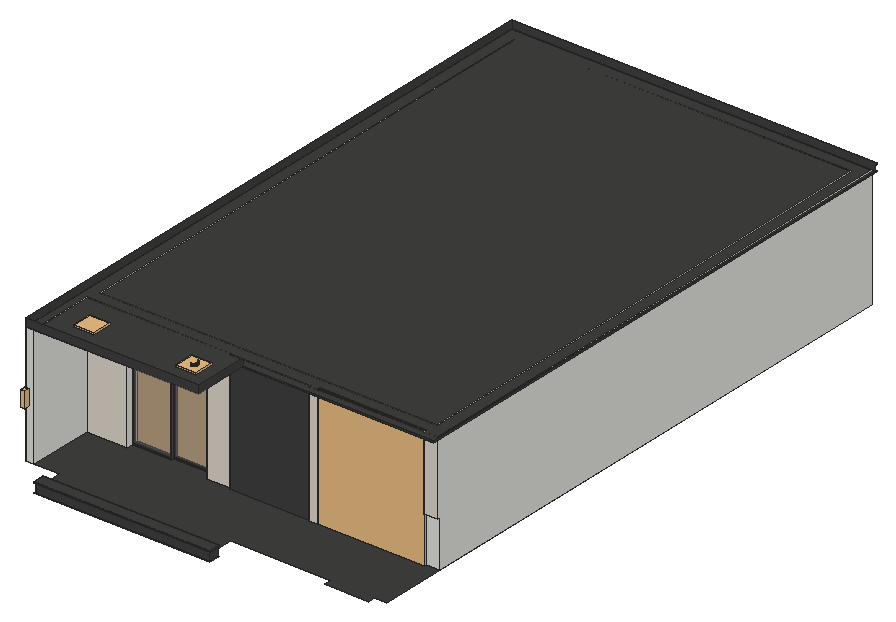
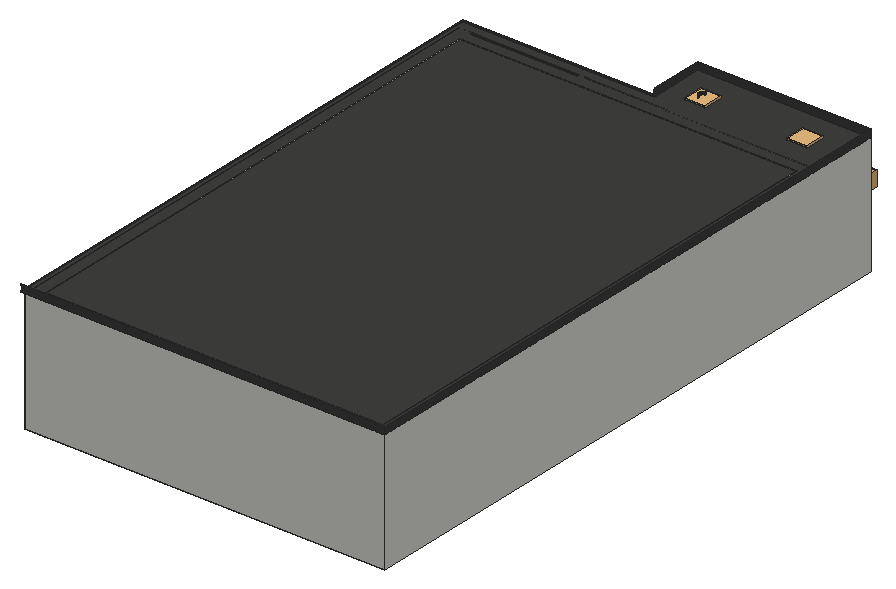
# SketchUp Ruby script. Lengths in inches.
U = 1.inch
M = Sketchup.active_model
def pt(a) = Geom::Point3d.new(a.map { |v| v * U })
def face(e, loops, mat)
  f = e.add_face(loops[0].map { |a| pt(a) })
  loops[1..].each { |l| e.add_face(l.map { |a| pt(a) }).erase! }
  f.material = f.back_material = mat if mat
  f
end
# faces: each face lists its corners as indices into pts; further lists are holes
def faces(e, pts, list, mat = nil) = list.each { |f| face(e, (f[0].is_a?(Array) ? f : [f]).map { |l| l.map { |i| pts[i] } }, mat) }
# xy, xz, yz: faces in a plane at the given z, y or x. An outline is a flat list of corners, or four numbers for a rectangle; further outlines are holes
def ring(l) = l.size == 4 ? [[l[0], l[1]], [l[2], l[1]], [l[2], l[3]], [l[0], l[3]]] : l.each_slice(2).to_a
def flat(e, list, mat, &to3) = list.each { |f| face(e, (f[0].is_a?(Array) ? f : [f]).map { |l| ring(l).map { |u, v| to3.(u, v) } }, mat) }
def xy(e, z, list, mat = nil) = flat(e, list, mat) { |x, y| [x, y, z] }
def xz(e, y, list, mat = nil) = flat(e, list, mat) { |x, z| [x, y, z] }
def yz(e, x, list, mat = nil) = flat(e, list, mat) { |y, z| [x, y, z] }
def lines(e, pts, list) = list.each { |a, b| e.add_line(pt(pts[a]), pt(pts[b])) }
# prism: a flat outline (further loops are holes) pulled along v
def prism(e, loops, v, mat = nil)
  f = face(e, loops, mat); d = Geom::Vector3d.new(v.map { |x| x * U })
  f.pushpull(f.normal.samedirection?(d) ? d.length : -d.length)
end
def box(e, o, s, mat = nil) = prism(e, [[o, [o[0] + s[0], o[1], o[2]], [o[0] + s[0], o[1] + s[1], o[2]], [o[0], o[1] + s[1], o[2]]]], [0, 0, s[2]], mat)
def at(x, y, z, deg = 0) = Geom::Transformation.translation(pt([x, y, z])) * Geom::Transformation.rotation(ORIGIN, Z_AXIS, deg.degrees)
def axes(o, x, y, z) = Geom::Transformation.new([*x, 0, *y, 0, *z, 0, *pt(o).to_a, 1])
def part(name) = M.definitions.add(name)
# library, detail: a bought-in or finely detailed component or shape, given as its bounding box
def library(name, o, s) = part(name).tap { |d| box(d.entities, o, s) }
def detail(e, o, s) = box(e.add_group.entities, o, s)
def put(e, d, t, mat = nil) = e.add_instance(d, t).tap { |i| i.material = mat if mat }
def group(e, t, mat = nil) = e.add_group.tap { |g| g.transformation = t; g.material = mat if mat }.entities
root = M.entities
M.materials.add("1448 AP 8253 RAVEN SONG").color = [64, 64, 63]
M.materials.add("[0135_DarkGray]").color = [81, 81, 81]
M.materials.add("[Stone Vein Gray]").color = [63, 63, 63]
M.materials.add("[Tile Various Tan]").color = [223, 216, 204]
M.materials.add("[Translucent Glass Gray]1").color = [128, 128, 128]
M.materials["[Translucent Glass Gray]1"].alpha = 0.15
c1 = part("PENTEK_RP Fineline 50S_Sliding_DoorCase_E1")
box(c1.entities,[0,0,0],[1.51,3.66,99.27],"[0135_DarkGray]")
c2 = part("PENTEK_RP Fineline 50S_SlidingDooe_Case_E2")
box(c2.entities,[0,0,0],[96.25,3.66,1.51],"[0135_DarkGray]")
c3 = part("pentek_RP Fineline 50S_SlidingDoor_Case")
put(c3.entities,c1,at(97.76,0,0))
put(c3.entities,c2,at(1.51,0,0))
put(c3.entities,c1,at(0,0,0))
put(c3.entities,c2,at(1.51,0,97.76))
c4 = part("PENTEK_RP Fineline 50S_SlidingDoor_GlazingBead_2")
box(c4.entities,[0,0,0],[0.56,0.59,94.39],"[0135_DarkGray]")
c5 = part("PENTEK_RP Fineline 50S_SlidingDoor_Glass")
box(c5.entities,[0,0,0],[46.58,0.16,94.39],"[Translucent Glass Gray]1")
c6 = part("PENTEK_RP Fineline 50S_SlidingDoor_GlazingBead")
box(c6.entities,[0,0,0],[45.47,0.59,0.56],"[0135_DarkGray]")
c7 = part("PENTEK_RP Fineline 50S_SlidingDoor_Leaf_E1")
xy(c7.entities,0,[[0,0,0.93,1.97],[0.93,1.57,1.49,1.97]],"[0135_DarkGray]")
xy(c7.entities,96.25,[[0,0,0.93,0,0.93,1.57,1.49,1.57,1.49,1.97,0,1.97]],"[0135_DarkGray]")
xz(c7.entities,0,[[0,0,0.93,96.25]],"[0135_DarkGray]")
xz(c7.entities,1.57,[[0.93,0,1.49,95.32],[0.93,95.32,1.49,96.25]],"[0135_DarkGray]")
xz(c7.entities,1.97,[[0,0,1.49,96.25]],"[0135_DarkGray]")
yz(c7.entities,0,[[0,0,1.97,96.25]],"[0135_DarkGray]")
yz(c7.entities,0.93,[[0,0,1.57,0.93],[0,0.93,1.57,95.32],[0,95.32,1.57,96.25]],"[0135_DarkGray]")
yz(c7.entities,1.49,[[1.57,0,1.97,95.32],[1.57,95.32,1.97,96.25]],"[0135_DarkGray]")
c8 = part("PENTEK_RP Fineline 50S_SlidingDoor_Leaf_E2")
xy(c8.entities,0,[[0,0,0,1.57,0.56,1.57,0.56,1.97,46.02,1.97,46.02,1.57,46.58,1.57,46.58,0]],"[0135_DarkGray]")
xy(c8.entities,0.93,[[0,0,46.58,1.57]],"[0135_DarkGray]")
xy(c8.entities,1.49,[[0.56,1.57,46.02,1.97]],"[0135_DarkGray]")
xz(c8.entities,0,[[0,0,46.58,0.93]],"[0135_DarkGray]")
xz(c8.entities,1.57,[[0,0,0.56,0.93],[46.02,0,46.58,0.93],[0.56,0.93,46.02,1.49]],"[0135_DarkGray]")
xz(c8.entities,1.97,[[0.56,0,46.02,1.49]],"[0135_DarkGray]")
yz(c8.entities,0,[[0,0,1.57,0.93]],"[0135_DarkGray]")
yz(c8.entities,0.56,[[1.57,0,1.97,0.93],[1.57,0.93,1.97,1.49]],"[0135_DarkGray]")
yz(c8.entities,46.02,[[1.57,0,1.97,0.93],[1.57,0.93,1.97,1.49]],"[0135_DarkGray]")
yz(c8.entities,46.58,[[0,0,1.57,0.93]],"[0135_DarkGray]")
c9 = part("PENTEK_RP Fineline S_SlidingDoor_Leaf1")
put(c9.entities,c4,at(0.93,0,0.93))
put(c9.entities,c4,at(46.96,0,0.93))
put(c9.entities,c5,at(1.49,1.42,0.93))
put(c9.entities,c6,at(1.49,0,0.93))
put(c9.entities,c5,at(1.49,0.59,0.93))
put(c9.entities,c7,at(0,0,0))
put(c9.entities,c7,axes([48.44,0,0],[-1,0,0],[0,1,0],[0,0,1]))
put(c9.entities,c8,axes([0.93,0,96.25],[1,0,0],[0,1,0],[0,0,-1]))
put(c9.entities,c8,at(0.93,0,0))
put(c9.entities,c6,at(1.49,0,94.77))
c10 = part("PENTEK_RP Fineline 50S_SlidingDoor_Leaf2")
put(c10.entities,c5,at(1.49,1.42,0.93))
put(c10.entities,c6,at(1.49,0,94.77))
put(c10.entities,c4,at(46.96,0,0.93))
put(c10.entities,c5,at(1.49,0.59,0.93))
put(c10.entities,c4,at(0.93,0,0.93))
put(c10.entities,c7,at(0,0,0))
put(c10.entities,c7,axes([48.44,0,0],[-1,0,0],[0,1,0],[0,0,1]))
put(c10.entities,c6,at(1.49,0,0.93))
put(c10.entities,c8,axes([0.93,0,96.25],[1,0,0],[0,1,0],[0,0,-1]))
put(c10.entities,c8,at(0.93,0,0))
c11 = part("PENTEK_RP+Fineline+50S_Sliding_Door (1)")
put(c11.entities,c3,at(0,-1.88,-0.09))
put(c11.entities,c9,at(1.51,-2.27,1.42))
put(c11.entities,c10,at(49.32,-0.3,1.42))
c12 = library("Group\#92",[0,0,0],[75.39,1.25,93])
c13 = library("Curtains",[0,0,0],[121.73,8.19,117.22])
c14 = library("WALL LIGHT 69",[4.19,4.05,-8.78],[4.61,5.7,17.13])
c15 = library("11",[-5.64,-5.64,-13.23],[15.28,15.28,13.23])
xy(root,373,[[31.93,174,167.89,174,167.89,183,166.86,183,166.86,175,32.96,175,32.96,183,31.93,183]],"1448 AP 8253 RAVEN SONG")
xy(root,375,[[39.29,221.5,39.21,221.51,39.14,221.52,38.9,221.55,38.83,221.57,38.75,221.58,38.67,221.6,38.6,221.625,38.52,221.65,38.45,221.67,38.3,221.73,38.16,221.79,38.09,221.83,38.02,221.86,37.88,221.94,37.82,221.98,37.75,222.03,37.6875,222.07,37.5,222.22,37.38,222.32,37.33,222.38,37.27,222.43,37.07,222.67,37.02,222.74,36.98,222.8,36.93,222.87,36.89,222.93,36.85,223,36.8125,223.07,36.78,223.14,36.74,223.21,36.65,223.42,36.62,223.5,36.6,223.57,36.57,223.65,36.55,223.72,36.53,223.8,36.52,223.875,36.5,223.95,36.48,224.11,36.47,224.1875,36.46,224.26,36.45,224.34,36.45,224.66,36.46,224.74,36.47,224.8125,36.48,224.89,36.5,225.05,36.52,225.125,36.53,225.2,36.55,225.28,36.57,225.35,36.6,225.43,36.62,225.5,36.65,225.58,36.74,225.79,36.78,225.86,36.8125,225.93,36.85,226,36.89,226.07,36.93,226.13,36.98,226.2,37.02,226.26,37.07,226.33,37.27,226.57,37.33,226.62,37.38,226.68,37.5,226.78,37.6875,226.93,37.75,226.97,37.82,227.02,37.88,227.06,38.02,227.14,38.09,227.17,38.16,227.21,38.3,227.27,38.45,227.33,38.52,227.35,38.6,227.375,38.67,227.4,38.75,227.42,38.83,227.43,38.9,227.45,39.14,227.48,39.21,227.49,39.29,227.5,39.61,227.5,39.69,227.49,39.76,227.48,40,227.45,40.07,227.43,40.15,227.42,40.23,227.4,40.3,227.375,40.38,227.35,40.45,227.33,40.53,227.3,40.74,227.21,40.8125,227.17,40.88,227.14,41.02,227.06,41.08,227.02,41.15,226.97,41.21,226.93,41.28,226.88,41.52,226.68,41.57,226.62,41.625,226.57,41.68,226.51,41.83,226.33,41.88,226.26,41.92,226.2,41.97,226.13,42.01,226.07,42.09,225.93,42.16,225.79,42.25,225.58,42.28,225.5,42.3,225.43,42.33,225.35,42.35,225.28,42.37,225.2,42.38,225.125,42.4,225.05,42.42,224.89,42.43,224.8125,42.44,224.74,42.45,224.66,42.45,224.34,42.44,224.26,42.43,224.1875,42.42,224.11,42.4,223.95,42.38,223.875,42.37,223.8,42.35,223.72,42.33,223.65,42.3,223.57,42.28,223.5,42.25,223.42,42.16,223.21,42.09,223.07,42.01,222.93,41.97,222.87,41.92,222.8,41.88,222.74,41.83,222.67,41.68,222.49,41.625,222.43,41.57,222.38,41.52,222.32,41.28,222.12,41.21,222.07,41.15,222.03,41.08,221.98,41.02,221.94,40.88,221.86,40.8125,221.83,40.74,221.79,40.53,221.7,40.45,221.67,40.38,221.65,40.3,221.625,40.23,221.6,40.15,221.58,40.07,221.57,40,221.55,39.76,221.52,39.69,221.51,39.61,221.5],[111.87,221.5,111.79,221.51,111.72,221.52,111.64,221.53,111.5625,221.54,111.48,221.55,111.41,221.57,111.33,221.58,111.25,221.6,111.18,221.625,111.1,221.65,111.03,221.67,110.95,221.7,110.74,221.79,110.67,221.83,110.6,221.86,110.46,221.94,110.4,221.98,110.33,222.03,110.27,222.07,110.2,222.12,109.96,222.32,109.91,222.38,109.85,222.43,109.65,222.67,109.6,222.74,109.56,222.8,109.51,222.87,109.47,222.93,109.39,223.07,109.36,223.14,109.32,223.21,109.23,223.42,109.2,223.5,109.18,223.57,109.15,223.65,109.13,223.72,109.11,223.8,109.1,223.875,109.08,223.95,109.06,224.11,109.05,224.1875,109.04,224.26,109.03,224.34,109.03,224.66,109.04,224.74,109.05,224.8125,109.06,224.89,109.08,225.05,109.1,225.125,109.11,225.2,109.13,225.28,109.15,225.35,109.18,225.43,109.2,225.5,109.23,225.58,109.32,225.79,109.36,225.86,109.39,225.93,109.47,226.07,109.51,226.13,109.56,226.2,109.6,226.26,109.65,226.33,109.85,226.57,109.91,226.62,109.96,226.68,110.2,226.88,110.27,226.93,110.33,226.97,110.4,227.02,110.46,227.06,110.6,227.14,110.67,227.17,110.74,227.21,110.95,227.3,111.03,227.33,111.1,227.35,111.18,227.375,111.25,227.4,111.33,227.42,111.41,227.43,111.48,227.45,111.5625,227.46,111.64,227.47,111.72,227.48,111.79,227.49,111.87,227.5,112.1875,227.5,112.27,227.49,112.34,227.48,112.58,227.45,112.65,227.43,112.73,227.42,112.81,227.4,112.88,227.375,112.96,227.35,113.03,227.33,113.11,227.3,113.32,227.21,113.39,227.17,113.46,227.14,113.6,227.06,113.66,227.02,113.73,226.97,113.79,226.93,113.86,226.88,114.1,226.68,114.15,226.62,114.21,226.57,114.26,226.51,114.3125,226.45,114.36,226.39,114.41,226.33,114.46,226.26,114.5,226.2,114.55,226.13,114.59,226.07,114.67,225.93,114.7,225.86,114.74,225.79,114.83,225.58,114.86,225.5,114.88,225.43,114.91,225.35,114.93,225.28,114.95,225.2,114.96,225.125,114.98,225.05,115,224.89,115.01,224.8125,115.02,224.74,115.03,224.66,115.03,224.34,115.02,224.26,115.01,224.1875,115,224.11,114.98,223.95,114.96,223.875,114.95,223.8,114.93,223.72,114.91,223.65,114.88,223.57,114.86,223.5,114.83,223.42,114.74,223.21,114.7,223.14,114.67,223.07,114.59,222.93,114.55,222.87,114.5,222.8,114.46,222.74,114.41,222.67,114.36,222.61,114.3125,222.55,114.26,222.49,114.21,222.43,114.15,222.38,114.1,222.32,113.86,222.12,113.79,222.07,113.73,222.03,113.66,221.98,113.6,221.94,113.46,221.86,113.39,221.83,113.32,221.79,113.11,221.7,113.03,221.67,112.96,221.65,112.88,221.625,112.81,221.6,112.73,221.58,112.65,221.57,112.58,221.55,112.34,221.52,112.27,221.51,112.1875,221.5],[184.45,221.5,184.3,221.52,184.14,221.54,184.0625,221.55,183.99,221.57,183.91,221.58,183.83,221.6,183.76,221.625,183.68,221.65,183.61,221.67,183.53,221.7,183.32,221.79,183.25,221.83,183.18,221.86,183.04,221.94,182.98,221.98,182.91,222.03,182.85,222.07,182.78,222.12,182.54,222.32,182.49,222.38,182.43,222.43,182.23,222.67,182.18,222.74,182.14,222.8,182.09,222.87,182.05,222.93,181.97,223.07,181.9375,223.14,181.9,223.21,181.81,223.42,181.78,223.5,181.76,223.57,181.73,223.65,181.71,223.72,181.69,223.8,181.68,223.875,181.66,223.95,181.64,224.11,181.625,224.1875,181.62,224.26,181.61,224.34,181.61,224.66,181.62,224.74,181.625,224.8125,181.64,224.89,181.66,225.05,181.68,225.125,181.69,225.2,181.71,225.28,181.73,225.35,181.76,225.43,181.78,225.5,181.81,225.58,181.9,225.79,181.9375,225.86,181.97,225.93,182.05,226.07,182.09,226.13,182.14,226.2,182.18,226.26,182.23,226.33,182.43,226.57,182.49,226.62,182.54,226.68,182.78,226.88,182.85,226.93,182.91,226.97,182.98,227.02,183.04,227.06,183.18,227.14,183.25,227.17,183.32,227.21,183.53,227.3,183.61,227.33,183.68,227.35,183.76,227.375,183.83,227.4,183.91,227.42,183.99,227.43,184.0625,227.45,184.14,227.46,184.3,227.48,184.45,227.5,184.77,227.5,184.85,227.49,184.92,227.48,185.16,227.45,185.23,227.43,185.31,227.42,185.39,227.4,185.46,227.375,185.54,227.35,185.61,227.33,185.69,227.3,185.9,227.21,185.97,227.17,186.04,227.14,186.18,227.06,186.24,227.02,186.31,226.97,186.375,226.93,186.5,226.83,186.68,226.68,186.73,226.62,186.79,226.57,186.99,226.33,187.04,226.26,187.08,226.2,187.125,226.13,187.17,226.07,187.25,225.93,187.28,225.86,187.32,225.79,187.41,225.58,187.4375,225.5,187.46,225.43,187.49,225.35,187.51,225.28,187.53,225.2,187.54,225.125,187.56,225.05,187.58,224.89,187.59,224.8125,187.6,224.74,187.61,224.66,187.61,224.34,187.6,224.26,187.59,224.1875,187.58,224.11,187.56,223.95,187.54,223.875,187.53,223.8,187.51,223.72,187.49,223.65,187.46,223.57,187.4375,223.5,187.41,223.42,187.32,223.21,187.28,223.14,187.25,223.07,187.17,222.93,187.125,222.87,187.08,222.8,187.04,222.74,186.99,222.67,186.79,222.43,186.73,222.38,186.68,222.32,186.5,222.17,186.375,222.07,186.31,222.03,186.24,221.98,186.18,221.94,186.04,221.86,185.97,221.83,185.9,221.79,185.69,221.7,185.61,221.67,185.54,221.65,185.46,221.625,185.39,221.6,185.31,221.58,185.23,221.57,185.16,221.55,184.92,221.52,184.85,221.51,184.77,221.5],[257.03,221.5,256.95,221.51,256.8,221.53,256.64,221.55,256.57,221.57,256.49,221.58,256.41,221.6,256.34,221.625,256.26,221.65,256.1875,221.67,256.11,221.7,255.9,221.79,255.83,221.83,255.76,221.86,255.62,221.94,255.56,221.98,255.49,222.03,255.43,222.07,255.36,222.12,255.18,222.27,255.125,222.32,255.07,222.38,255.01,222.43,254.81,222.67,254.76,222.74,254.72,222.8,254.67,222.87,254.63,222.93,254.55,223.07,254.52,223.14,254.48,223.21,254.39,223.42,254.36,223.5,254.34,223.57,254.3125,223.65,254.29,223.72,254.27,223.8,254.26,223.875,254.24,223.95,254.22,224.11,254.21,224.1875,254.2,224.26,254.19,224.34,254.19,224.66,254.2,224.74,254.21,224.8125,254.22,224.89,254.24,225.05,254.26,225.125,254.27,225.2,254.29,225.28,254.3125,225.35,254.34,225.43,254.36,225.5,254.39,225.58,254.48,225.79,254.52,225.86,254.55,225.93,254.63,226.07,254.67,226.13,254.72,226.2,254.76,226.26,254.81,226.33,255.01,226.57,255.07,226.62,255.125,226.68,255.18,226.73,255.36,226.88,255.43,226.93,255.49,226.97,255.56,227.02,255.62,227.06,255.76,227.14,255.83,227.17,255.9,227.21,256.11,227.3,256.1875,227.33,256.26,227.35,256.34,227.375,256.41,227.4,256.49,227.42,256.57,227.43,256.64,227.45,256.8,227.47,256.95,227.49,257.03,227.5,257.35,227.5,257.43,227.49,257.5,227.48,257.74,227.45,257.8125,227.43,257.89,227.42,257.97,227.4,258.04,227.375,258.12,227.35,258.19,227.33,258.27,227.3,258.48,227.21,258.55,227.17,258.62,227.14,258.76,227.06,258.82,227.02,258.89,226.97,258.95,226.93,259.02,226.88,259.26,226.68,259.3125,226.62,259.37,226.57,259.57,226.33,259.62,226.26,259.66,226.2,259.71,226.13,259.75,226.07,259.83,225.93,259.86,225.86,259.9,225.79,259.99,225.58,260.02,225.5,260.04,225.43,260.07,225.35,260.09,225.28,260.11,225.2,260.14,225.05,260.16,224.89,260.17,224.8125,260.18,224.74,260.1875,224.66,260.1875,224.58,260.19,224.5,260.1875,224.42,260.1875,224.34,260.18,224.26,260.17,224.1875,260.16,224.11,260.14,223.95,260.11,223.8,260.09,223.72,260.07,223.65,260.04,223.57,260.02,223.5,259.99,223.42,259.9,223.21,259.86,223.14,259.83,223.07,259.75,222.93,259.71,222.87,259.66,222.8,259.62,222.74,259.57,222.67,259.37,222.43,259.3125,222.38,259.26,222.32,259.02,222.12,258.95,222.07,258.89,222.03,258.82,221.98,258.76,221.94,258.62,221.86,258.55,221.83,258.48,221.79,258.27,221.7,258.19,221.67,258.12,221.65,258.04,221.625,257.97,221.6,257.89,221.58,257.8125,221.57,257.74,221.55,257.5,221.52,257.43,221.51,257.35,221.5]],"1448 AP 8253 RAVEN SONG")
xy(root,378,[[35.02,183,166.86,183,166.86,195,244.11,195,244.11,189,278.1,189,278.1,195,287.37,195,287.37,663,9.27,663,9.27,195,35.02,195]],"1448 AP 8253 RAVEN SONG")
xy(root,380,[[31.93,174,31.93,183,32.96,183,32.96,175,167.89,175,167.89,174],[166.86,175,167.89,183]],"1448 AP 8253 RAVEN SONG")
xy(root,381,[[31.93,174,167.89,183]],"1448 AP 8253 RAVEN SONG")
xy(root,471,[[[9.27,195,9.27,663,290.46,663,290.46,237,142.14,237,142.14,195],[39.3,217.5,39.62,217.5,39.7,217.51,39.77,217.52,40.01,217.55,40.08,217.57,40.24,217.61,40.3125,217.625,40.39,217.65,40.46,217.68,40.54,217.7,40.68,217.76,40.75,217.8,40.82,217.83,41.03,217.95,41.09,217.99,41.16,218.03,41.22,218.08,41.29,218.125,41.35,218.18,41.47,218.28,41.63,218.44,41.6875,218.5,41.74,218.56,41.84,218.68,41.88,218.75,41.93,218.81,42.01,218.94,42.13,219.15,42.16,219.22,42.2,219.29,42.23,219.36,42.25,219.4375,42.28,219.51,42.31,219.58,42.33,219.66,42.35,219.73,42.37,219.8125,42.39,219.89,42.4,219.96,42.41,220.04,42.43,220.12,42.43,220.2,42.44,220.28,42.45,220.35,42.45,220.67,42.44,220.75,42.43,220.82,42.4,221.06,42.38,221.13,42.34,221.29,42.32,221.36,42.3,221.4375,42.27,221.51,42.25,221.59,42.22,221.66,42.1875,221.73,42.15,221.8,42.12,221.87,42,222.08,41.96,222.14,41.92,222.21,41.87,222.27,41.82,222.34,41.67,222.52,41.62,222.57,41.5625,222.63,41.51,222.68,41.45,222.74,41.27,222.89,41.2,222.93,41.14,222.98,41.07,223.02,41.01,223.0625,40.94,223.1,40.8,223.18,40.73,223.21,40.66,223.25,40.59,223.28,40.51,223.3,40.37,223.36,40.29,223.38,40.22,223.4,40.14,223.42,40.0625,223.4375,39.99,223.45,39.91,223.46,39.83,223.48,39.75,223.48,39.67,223.49,39.6,223.5,39.28,223.5,39.2,223.49,39.05,223.47,38.89,223.45,38.82,223.43,38.66,223.39,38.59,223.375,38.51,223.35,38.4375,223.32,38.36,223.3,38.22,223.24,38.15,223.2,38.08,223.17,37.87,223.05,37.81,223.01,37.74,222.97,37.68,222.92,37.61,222.875,37.55,222.82,37.43,222.72,37.375,222.67,37.32,222.61,37.21,222.5,37.11,222.38,37.0625,222.32,37.02,222.25,36.97,222.19,36.89,222.06,36.77,221.85,36.74,221.78,36.7,221.71,36.67,221.64,36.65,221.5625,36.62,221.49,36.59,221.42,36.57,221.34,36.55,221.27,36.53,221.1875,36.51,221.11,36.5,221.04,36.49,220.96,36.47,220.88,36.47,220.8,36.46,220.72,36.45,220.65,36.45,220.33,36.46,220.25,36.47,220.18,36.5,219.94,36.52,219.87,36.56,219.71,36.58,219.64,36.6,219.5625,36.625,219.49,36.65,219.41,36.71,219.27,36.75,219.2,36.78,219.13,36.9,218.92,36.94,218.86,36.98,218.79,37.03,218.73,37.08,218.66,37.125,218.6,37.18,218.54,37.23,218.48,37.45,218.26,37.63,218.11,37.7,218.07,37.76,218.02,37.83,217.98,37.89,217.9375,37.96,217.9,38.1,217.82,38.17,217.79,38.24,217.75,38.3125,217.72,38.39,217.7,38.53,217.64,38.61,217.62,38.68,217.6,38.76,217.58,38.84,217.5625,38.91,217.55,38.99,217.54,39.07,217.52,39.15,217.52,39.23,217.51],[117.99,217.5,118.31,217.5,118.39,217.51,118.46,217.52,118.7,217.55,118.77,217.57,118.93,217.61,119,217.625,119.08,217.65,119.15,217.68,119.23,217.7,119.37,217.76,119.44,217.8,119.51,217.83,119.72,217.95,119.78,217.99,119.85,218.03,119.91,218.08,119.98,218.125,120.04,218.18,120.16,218.28,120.38,218.5,120.53,218.68,120.57,218.75,120.62,218.81,120.7,218.94,120.82,219.15,120.85,219.22,120.89,219.29,120.92,219.36,120.94,219.4375,120.97,219.51,121,219.58,121.02,219.66,121.04,219.73,121.06,219.8125,121.08,219.89,121.09,219.96,121.1,220.04,121.12,220.12,121.13,220.28,121.14,220.35,121.14,220.67,121.13,220.75,121.12,220.82,121.09,221.06,121.07,221.13,121.03,221.29,121.01,221.36,120.99,221.4375,120.96,221.51,120.9375,221.59,120.91,221.66,120.84,221.8,120.81,221.87,120.69,222.08,120.65,222.14,120.61,222.21,120.56,222.27,120.51,222.34,120.36,222.52,120.14,222.74,119.96,222.89,119.89,222.93,119.83,222.98,119.76,223.02,119.7,223.0625,119.63,223.1,119.5625,223.14,119.49,223.18,119.42,223.21,119.35,223.25,119.28,223.28,119.2,223.3,119.06,223.36,118.98,223.38,118.91,223.4,118.83,223.42,118.75,223.4375,118.68,223.45,118.6,223.46,118.52,223.48,118.44,223.48,118.36,223.49,118.29,223.5,117.97,223.5,117.89,223.49,117.82,223.48,117.58,223.45,117.51,223.43,117.35,223.39,117.28,223.375,117.2,223.35,117.13,223.32,117.05,223.3,116.91,223.24,116.84,223.2,116.77,223.17,116.63,223.09,116.5625,223.05,116.5,223.01,116.43,222.97,116.37,222.92,116.3,222.875,116.24,222.82,116.18,222.77,116.07,222.67,115.9,222.5,115.75,222.32,115.71,222.25,115.66,222.19,115.58,222.06,115.46,221.85,115.43,221.78,115.39,221.71,115.36,221.64,115.34,221.5625,115.31,221.49,115.28,221.42,115.26,221.34,115.24,221.27,115.22,221.1875,115.2,221.11,115.1875,221.04,115.18,220.96,115.16,220.88,115.16,220.8,115.15,220.72,115.14,220.65,115.14,220.33,115.15,220.25,115.16,220.18,115.19,219.94,115.21,219.87,115.25,219.71,115.27,219.64,115.29,219.5625,115.32,219.49,115.34,219.41,115.4,219.27,115.4375,219.2,115.47,219.13,115.59,218.92,115.63,218.86,115.67,218.79,115.72,218.73,115.77,218.66,115.92,218.48,116.14,218.26,116.32,218.11,116.39,218.07,116.45,218.02,116.52,217.98,116.58,217.9375,116.65,217.9,116.79,217.82,116.86,217.79,116.93,217.75,117,217.72,117.08,217.7,117.22,217.64,117.3,217.62,117.45,217.58,117.53,217.5625,117.6,217.55,117.68,217.54,117.76,217.52,117.84,217.52,117.92,217.51]]],"1448 AP 8253 RAVEN SONG")
xz(root,174,[[31.93,380,167.89,381]],"1448 AP 8253 RAVEN SONG")
xz(root,175,[[32.96,373,166.86,380]],"1448 AP 8253 RAVEN SONG")
xz(root,183,[[32.96,378,32.96,380,31.93,380,31.93,381,167.89,381,167.89,380,166.86,380,166.86,378]],"1448 AP 8253 RAVEN SONG")
xz(root,195,[[9.27,471,142.14,477]],"1448 AP 8253 RAVEN SONG")
xz(root,217.5,[[118.23,471,118.31,474]],"1448 AP 8253 RAVEN SONG")
xz(root,237,[[142.14,471,290.46,472]],"1448 AP 8253 RAVEN SONG")
xz(root,663,[[9.27,471,9.27,477,290.46,477,290.46,476,289.43,476,289.43,472,290.46,472,290.46,471]],"1448 AP 8253 RAVEN SONG")
yz(root,9.27,[[195,471,663,477]],"1448 AP 8253 RAVEN SONG")
yz(root,31.93,[[174,380,183,381]],"1448 AP 8253 RAVEN SONG")
yz(root,32.96,[[175,373,183,380]],"1448 AP 8253 RAVEN SONG")
yz(root,121.14,[[220.35,471,220.43,474],[220.43,471,220.51,474],[220.51,471,220.59,474],[220.59,471,220.67,474]],"1448 AP 8253 RAVEN SONG")
yz(root,142.14,[[195,471,237,471,237,472,238,472,238,476,237,476,237,477,195,477]],"1448 AP 8253 RAVEN SONG")
yz(root,166.86,[[175,373,183,380]],"1448 AP 8253 RAVEN SONG")
yz(root,167.89,[[174,380,183,381]],"1448 AP 8253 RAVEN SONG")
yz(root,290.46,[[237,471,663,472]],"1448 AP 8253 RAVEN SONG")
p = [[118.39,217.51,471],[118.31,217.5,471],[118.31,217.5,474],[118.39,217.51,474],[118.46,217.52,471],[118.46,217.52,474],
  [118.62,217.54,471],[118.54,217.53,471],[118.54,217.53,474],[118.62,217.54,474],[118.7,217.55,471],[118.7,217.55,474],
  [118.77,217.57,471],[118.77,217.57,474],[118.85,217.59,471],[118.85,217.59,474],[119,217.625,471],[118.93,217.61,471],
  [118.93,217.61,474],[119,217.625,474],[119.08,217.65,471],[119.08,217.65,474],[119.15,217.68,471],[119.15,217.68,474],
  [119.3,217.73,471],[119.23,217.7,471],[119.23,217.7,474],[119.3,217.73,474],[119.37,217.76,471],[119.37,217.76,474],
  [119.51,217.83,471],[119.44,217.8,471],[119.44,217.8,474],[119.51,217.83,474],[119.58,217.87,471],[119.58,217.87,474],
  [119.72,217.95,471],[119.65,217.91,471],[119.65,217.91,474],[119.72,217.95,474],[119.78,217.99,471],[119.78,217.99,474],
  [119.91,218.08,471],[119.85,218.03,471],[119.85,218.03,474],[119.91,218.08,474],[119.98,218.125,471],[119.98,218.125,474],
  [120.04,218.18,471],[120.04,218.18,474],[120.1,218.23,471],[120.1,218.23,474],[120.16,218.28,471],[120.16,218.28,474],
  [120.27,218.39,471],[120.21,218.33,471],[120.21,218.33,474],[120.27,218.39,474],[120.38,218.5,471],[120.32,218.44,471],
  [120.32,218.44,474],[120.38,218.5,474],[120.43,218.56,471],[120.43,218.56,474],[120.48,218.62,471],[120.48,218.62,474],
  [120.53,218.68,471],[120.53,218.68,474],[120.57,218.75,471],[120.57,218.75,474],[120.62,218.81,471],[120.62,218.81,474],
  [120.66,218.875,471],[120.66,218.875,474],[120.74,219.01,471],[120.7,218.94,471],[120.7,218.94,474],[120.74,219.01,474],
  [120.78,219.08,471],[120.78,219.08,474],[120.85,219.22,471],[120.82,219.15,471],[120.82,219.15,474],[120.85,219.22,474],
  [120.89,219.29,471],[120.89,219.29,474],[120.92,219.36,471],[120.92,219.36,474],[120.97,219.51,471],[120.94,219.4375,471],
  [120.94,219.4375,474],[120.97,219.51,474],[121,219.58,471],[121,219.58,474],[121.02,219.66,471],[121.02,219.66,474],
  [121.06,219.8125,471],[121.04,219.73,471],[121.04,219.73,474],[121.06,219.8125,474],[121.08,219.89,471],[121.08,219.89,474],
  [121.09,219.96,471],[121.09,219.96,474],[121.12,220.12,471],[121.1,220.04,471],[121.1,220.04,474],[121.12,220.12,474],
  [121.125,220.2,471],[121.125,220.2,474],[121.13,220.28,471],[121.13,220.28,474],[121.14,220.35,471],[121.14,220.35,474],
  [121.12,220.82,471],[121.13,220.75,471],[121.13,220.75,474],[121.12,220.82,474],[121.14,220.67,471],[121.14,220.67,474],
  [121.11,220.9,471],[121.11,220.9,474],[121.1,220.98,471],[121.1,220.98,474],[121.09,221.06,471],[121.09,221.06,474],
  [121.05,221.21,471],[121.07,221.13,471],[121.07,221.13,474],[121.05,221.21,474],[121.03,221.29,471],[121.03,221.29,474],
  [121.01,221.36,471],[121.01,221.36,474],[120.96,221.51,471],[120.99,221.4375,471],[120.99,221.4375,474],[120.96,221.51,474],
  [120.9375,221.59,471],[120.9375,221.59,474],[120.91,221.66,471],[120.91,221.66,474],[120.84,221.8,471],[120.875,221.73,471],
  [120.875,221.73,474],[120.84,221.8,474],[120.81,221.87,471],[120.81,221.87,474],[120.73,222.01,471],[120.77,221.94,471],
  [120.77,221.94,474],[120.73,222.01,474],[120.69,222.08,471],[120.69,222.08,474],[120.61,222.21,471],[120.65,222.14,471],
  [120.65,222.14,474],[120.61,222.21,474],[120.56,222.27,471],[120.56,222.27,474],[120.46,222.4,471],[120.51,222.34,471],
  [120.51,222.34,474],[120.46,222.4,474],[120.41,222.46,471],[120.41,222.46,474],[120.31,222.57,471],[120.36,222.52,471],
  [120.36,222.52,474],[120.31,222.57,474],[120.2,222.68,471],[120.25,222.63,471],[120.25,222.63,474],[120.2,222.68,474],
  [120.08,222.79,471],[120.14,222.74,471],[120.14,222.74,474],[120.08,222.79,474],[119.96,222.89,471],[120.02,222.84,471],
  [120.02,222.84,474],[119.96,222.89,474],[119.83,222.98,471],[119.89,222.93,471],[119.89,222.93,474],[119.83,222.98,474],
  [119.7,223.0625,471],[119.76,223.02,471],[119.76,223.02,474],[119.7,223.0625,474],[119.49,223.18,471],[119.5625,223.14,471],
  [119.5625,223.14,474],[119.49,223.18,474],[119.63,223.1,471],[119.63,223.1,474]]
faces(root,p,[[0,1,2,3],[4,0,3,5],[6,7,8,9],[7,4,5,8],[10,6,9,11],[12,10,11,13],[14,12,13,15],[16,17,18,19],
  [17,14,15,18],[20,16,19,21],[22,20,21,23],[24,25,26,27],[25,22,23,26],[28,24,27,29],[30,31,32,33],[31,28,29,32],
  [34,30,33,35],[36,37,38,39],[37,34,35,38],[40,36,39,41],[42,43,44,45],[43,40,41,44],[46,42,45,47],[48,46,47,49],
  [50,48,49,51],[52,50,51,53],[54,55,56,57],[55,52,53,56],[58,59,60,61],[59,54,57,60],[62,58,61,63],[64,62,63,65],
  [66,64,65,67],[68,66,67,69],[70,68,69,71],[72,70,71,73],[74,75,76,77],[75,72,73,76],[78,74,77,79],[80,81,82,83],
  [81,78,79,82],[84,80,83,85],[86,84,85,87],[88,89,90,91],[89,86,87,90],[92,88,91,93],[94,92,93,95],[96,97,98,99],
  [97,94,95,98],[100,96,99,101],[102,100,101,103],[104,105,106,107],[105,102,103,106],[108,104,107,109],[110,108,109,111],[112,110,111,113],
  [114,115,116,117],[115,118,119,116],[120,114,117,121],[122,120,121,123],[124,122,123,125],[126,127,128,129],[127,124,125,128],[130,126,129,131],
  [132,130,131,133],[134,135,136,137],[135,132,133,136],[138,134,137,139],[140,138,139,141],[142,143,144,145],[143,140,141,144],[146,142,145,147],
  [148,149,150,151],[149,146,147,150],[152,148,151,153],[154,155,156,157],[155,152,153,156],[158,154,157,159],[160,161,162,163],[161,158,159,162],
  [164,160,163,165],[166,167,168,169],[167,164,165,168],[170,171,172,173],[171,166,169,172],[174,175,176,177],[175,170,173,176],[178,179,180,181],
  [179,174,177,180],[182,183,184,185],[183,178,181,184],[186,187,188,189],[187,182,185,188],[190,191,192,193],[191,194,195,192],[194,186,189,195]],"1448 AP 8253 RAVEN SONG")
put(root,c11,axes([44.99,253.22,376.61],[0.63625,0,0],[0,1,0],[0,0,0.80042]))
g1 = group(root,at(9.27,195,378))
xy(g1,0,[[0,0,0,468,278.1,468,278.1,51,185.4,51,185.4,49,179.22,49,179.22,50,117.42,50,117.42,51,98.88,51,98.88,60,268.83,60,268.83,459,9.27,459,9.27,60,37.08,60,37.08,51,6.18,51,6.18,0]])
xy(g1,36,[[267.8,49,278.1,51]])
xy(g1,78,[[37.08,51,98.88,60]])
xy(g1,93,[[[0,0,6.18,0,6.18,51,117.42,51,117.42,50,179.22,50,179.22,49,185.4,49,185.4,51,267.8,51,267.8,49,278.1,49,278.1,468,0,468],[9.27,60,268.83,459]]])
xz(g1,0,[[0,0,6.18,93]])
xz(g1,49,[[179.22,0,185.4,93],[267.8,36,278.1,93]],"[Tile Various Tan]")
xz(g1,50,[[117.42,0,179.22,93]],"[Stone Vein Gray]")
xz(g1,51,[[185.4,0,278.1,0,278.1,36,267.8,36,267.8,93,185.4,93]])
xz(g1,51,[[6.18,0,37.08,0,37.08,78,98.88,78,98.88,0,117.42,0,117.42,93,6.18,93]],"[Tile Various Tan]")
xz(g1,60,[[9.27,0,9.27,93,268.83,93,268.83,0,98.88,0,98.88,78,37.08,78,37.08,0]])
xz(g1,459,[[9.27,0,268.83,93]])
xz(g1,468,[[0,0,278.1,93]])
yz(g1,0,[[0,0,468,93]])
yz(g1,6.18,[[0,0,51,93]])
yz(g1,9.27,[[60,0,459,93]])
yz(g1,37.08,[[51,0,60,78]])
yz(g1,98.88,[[51,0,60,78]])
yz(g1,117.42,[[50,0,51,93]])
yz(g1,179.22,[[49,0,50,93]])
yz(g1,185.4,[[49,0,51,93]])
yz(g1,267.8,[[49,36,51,93]])
yz(g1,268.83,[[60,0,459,93]])
yz(g1,278.1,[[51,0,468,0,468,93,49,93,49,36,51,36]])
put(g1,c12,axes([185.4,49.5,0],[1.09303,0,0],[0,1,0],[0,0,1]))
put(root,c13,axes([31.72,255,378.94],[0.721,0,0],[0,0.7,0],[0,0,0.7]))
put(root,c14,axes([15.53,175.18,432.14],[0.7,0,0],[0,0.7,0],[0,0,0.7]))
put(root,c15,at(37.45,218.5,472.25),"1448 AP 8253 RAVEN SONG")
put(root,c15,at(116.14,218.5,472.25),"1448 AP 8253 RAVEN SONG")
